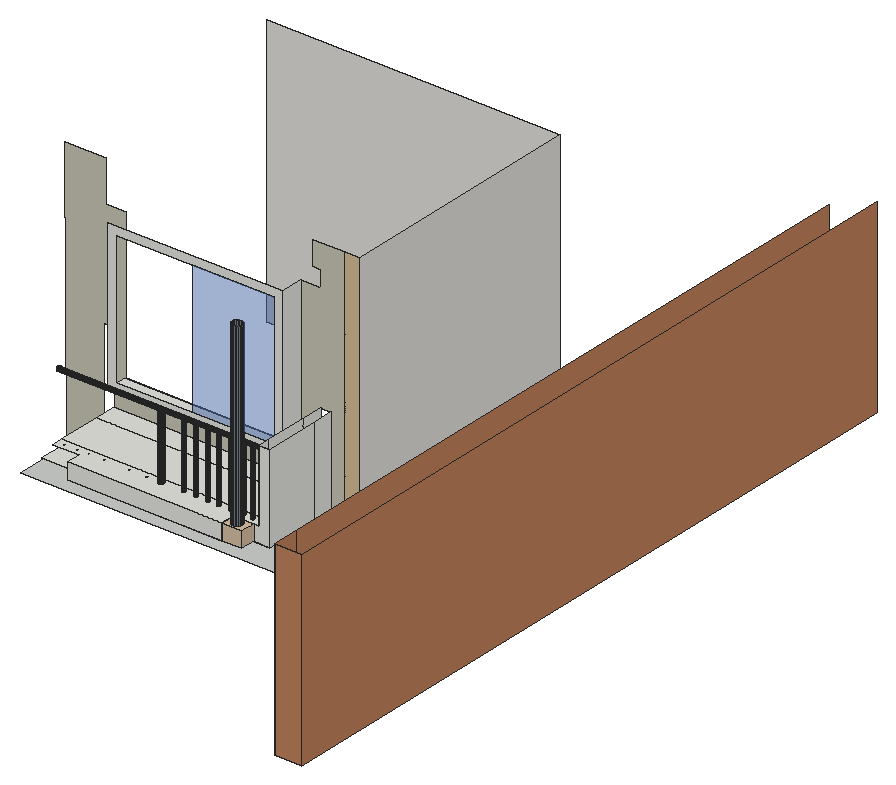
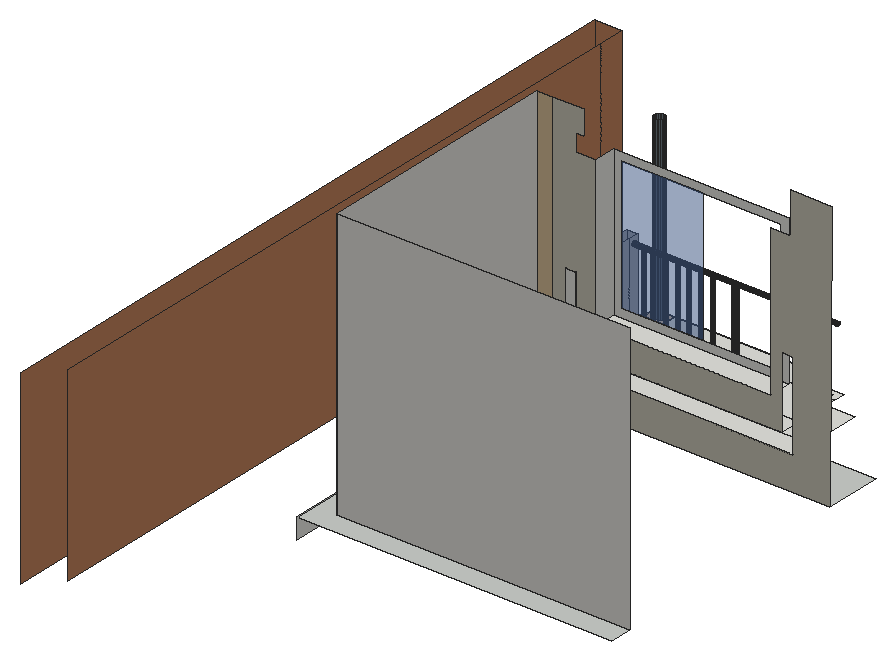
# SketchUp Ruby script. Lengths in inches.
U = 1.inch
M = Sketchup.active_model
def pt(a) = Geom::Point3d.new(a.map { |v| v * U })
def face(e, loops, mat)
  f = e.add_face(loops[0].map { |a| pt(a) })
  loops[1..].each { |l| e.add_face(l.map { |a| pt(a) }).erase! }
  f.material = f.back_material = mat if mat
  f
end
# faces: each face lists its corners as indices into pts; further lists are holes
def faces(e, pts, list, mat = nil) = list.each { |f| face(e, (f[0].is_a?(Array) ? f : [f]).map { |l| l.map { |i| pts[i] } }, mat) }
# xy, xz, yz: faces in a plane at the given z, y or x. An outline is a flat list of corners, or four numbers for a rectangle; further outlines are holes
def ring(l) = l.size == 4 ? [[l[0], l[1]], [l[2], l[1]], [l[2], l[3]], [l[0], l[3]]] : l.each_slice(2).to_a
def flat(e, list, mat, &to3) = list.each { |f| face(e, (f[0].is_a?(Array) ? f : [f]).map { |l| ring(l).map { |u, v| to3.(u, v) } }, mat) }
def xy(e, z, list, mat = nil) = flat(e, list, mat) { |x, y| [x, y, z] }
def xz(e, y, list, mat = nil) = flat(e, list, mat) { |x, z| [x, y, z] }
def yz(e, x, list, mat = nil) = flat(e, list, mat) { |y, z| [x, y, z] }
def lines(e, pts, list) = list.each { |a, b| e.add_line(pt(pts[a]), pt(pts[b])) }
# prism: a flat outline (further loops are holes) pulled along v
def prism(e, loops, v, mat = nil)
  f = face(e, loops, mat); d = Geom::Vector3d.new(v.map { |x| x * U })
  f.pushpull(f.normal.samedirection?(d) ? d.length : -d.length)
end
def box(e, o, s, mat = nil) = prism(e, [[o, [o[0] + s[0], o[1], o[2]], [o[0] + s[0], o[1] + s[1], o[2]], [o[0], o[1] + s[1], o[2]]]], [0, 0, s[2]], mat)
def at(x, y, z, deg = 0) = Geom::Transformation.translation(pt([x, y, z])) * Geom::Transformation.rotation(ORIGIN, Z_AXIS, deg.degrees)
def axes(o, x, y, z) = Geom::Transformation.new([*x, 0, *y, 0, *z, 0, *pt(o).to_a, 1])
def part(name) = M.definitions.add(name)
# library, detail: a bought-in or finely detailed component or shape, given as its bounding box
def library(name, o, s) = part(name).tap { |d| box(d.entities, o, s) }
def detail(e, o, s) = box(e.add_group.entities, o, s)
def put(e, d, t, mat = nil) = e.add_instance(d, t).tap { |i| i.material = mat if mat }
def group(e, t, mat = nil) = e.add_group.tap { |g| g.transformation = t; g.material = mat if mat }.entities
root = M.entities
M.materials.add("[Basic Tile]").color = [203, 206, 202]
M.materials.add("[Formica Beige]").color = [211, 187, 149]
M.materials.add("[Formica Graystone]").color = [198, 194, 180]
M.materials.add("[Formica Laminate Dark]").color = [50, 53, 60]
M.materials.add("[Formica Laminate Light]").color = [213, 189, 164]
M.materials.add("[Formica Speckled Grey]").color = [112, 125, 132]
M.materials.add("[Terrazzo Tile Accent]").color = [224, 221, 217]
M.materials.add("[Translucent Glass Blue]").color = [85, 126, 201]
M.materials["[Translucent Glass Blue]"].alpha = 0.5
M.materials.add("[Wood Veneer 02]").color = [190, 128, 91]
xy(root,9,[[271.94,88.35,402.13,114.1],[402.13,88.35,411.85,88.35,411.85,235.11,271.94,235.11,271.94,225.39,402.13,225.39]],"[Basic Tile]")
xy(root,24.1875,[[304.9375,73.57,304.9375,80.01,288.3125,80.01,288.3125,104.39,389.375,104.39,389.375,80.01,373.41,80.01,373.41,73.57],[288.3125,104.39,389.375,114.1]])
xy(root,24.1875,[[373.41,73.57,382.25,80.01]],"[Formica Laminate Light]")
xy(root,31.3,[[[304.9375,73.57,373.41,73.57,373.41,80.01,384.76,80.01,384.76,84.92,293.16,84.92,293.16,80.01,304.9375,80.01],[339.03,81.65,338.7,81.69,338.4,81.82,338.14,82.02,337.94,82.27,337.82,82.58,337.78,82.9,337.82,83.22,337.94,83.52,338.14,83.78,338.4,83.98,338.7,84.11,339.03,84.15,339.35,84.11,339.65,83.98,339.91,83.78,340.11,83.52,340.23,83.22,340.28,82.9,340.23,82.58,340.11,82.27,339.91,82.02,339.65,81.82,339.35,81.69],[349.03,81.89,348.85,81.92,348.68,81.98,348.54,82.09,348.43,82.24,348.36,82.4,348.34,82.58,348.36,82.76,348.43,82.92,348.54,83.07,348.68,83.18,348.85,83.24,349.03,83.27,349.21,83.24,349.37,83.18,349.51,83.07,349.625,82.92,349.69,82.76,349.72,82.58,349.69,82.4,349.625,82.24,349.51,82.09,349.37,81.98,349.21,81.92],[379.9,81.89,379.73,81.92,379.56,81.98,379.42,82.09,379.31,82.24,379.24,82.4,379.22,82.58,379.24,82.76,379.31,82.92,379.42,83.07,379.56,83.18,379.73,83.24,379.9,83.27,380.08,83.24,380.25,83.18,380.39,83.07,380.5,82.92,380.57,82.76,380.59,82.58,380.57,82.4,380.5,82.24,380.39,82.09,380.25,81.98,380.08,81.92],[354.6875,81.89,354.51,81.92,354.35,81.98,354.2,82.09,354.09,82.24,354.02,82.4,354,82.58,354.02,82.76,354.09,82.92,354.2,83.07,354.35,83.18,354.51,83.24,354.6875,83.27,354.87,83.24,355.03,83.18,355.18,83.07,355.28,82.92,355.35,82.76,355.375,82.58,355.35,82.4,355.28,82.24,355.18,82.09,355.03,81.98,354.87,81.92],[375.8125,81.89,375.64,81.92,375.47,81.98,375.33,82.09,375.22,82.24,375.15,82.4,375.125,82.58,375.15,82.76,375.22,82.92,375.33,83.07,375.47,83.18,375.64,83.24,375.8125,83.27,375.99,83.24,376.16,83.18,376.3,83.07,376.41,82.92,376.48,82.76,376.5,82.58,376.48,82.4,376.41,82.24,376.3,82.09,376.16,81.98,375.99,81.92],[359.9375,81.89,359.76,81.92,359.6,81.98,359.45,82.09,359.34,82.24,359.27,82.4,359.25,82.58,359.27,82.76,359.34,82.92,359.45,83.07,359.6,83.18,359.76,83.24,359.9375,83.27,360.12,83.24,360.28,83.18,360.43,83.07,360.53,82.92,360.6,82.76,360.625,82.58,360.6,82.4,360.53,82.24,360.43,82.09,360.28,81.98,360.12,81.92],[370.25,81.89,370.07,81.92,369.91,81.98,369.77,82.09,369.66,82.24,369.59,82.4,369.5625,82.58,369.59,82.76,369.66,82.92,369.77,83.07,369.91,83.18,370.07,83.24,370.25,83.27,370.43,83.24,370.6,83.18,370.74,83.07,370.85,82.92,370.92,82.76,370.9375,82.58,370.92,82.4,370.85,82.24,370.74,82.09,370.6,81.98,370.43,81.92],[364.8125,81.89,364.64,81.92,364.47,81.98,364.33,82.09,364.22,82.24,364.15,82.4,364.125,82.58,364.15,82.76,364.22,82.92,364.33,83.07,364.47,83.18,364.64,83.24,364.8125,83.27,364.99,83.24,365.16,83.18,365.3,83.07,365.41,82.92,365.48,82.76,365.5,82.58,365.48,82.4,365.41,82.24,365.3,82.09,365.16,81.98,364.99,81.92],[332.6875,81.89,332.51,81.92,332.35,81.98,332.2,82.09,332.09,82.24,332.02,82.4,332,82.58,332.02,82.76,332.09,82.92,332.2,83.07,332.35,83.18,332.51,83.24,332.6875,83.27,332.87,83.24,333.03,83.18,333.18,83.07,333.28,82.92,333.35,82.76,333.375,82.58,333.35,82.4,333.28,82.24,333.18,82.09,333.03,81.98,332.87,81.92],[296.0625,81.89,295.89,81.92,295.72,81.98,295.58,82.09,295.47,82.24,295.4,82.4,295.375,82.58,295.4,82.76,295.47,82.92,295.58,83.07,295.72,83.18,295.89,83.24,296.0625,83.27,296.24,83.24,296.41,83.18,296.55,83.07,296.66,82.92,296.73,82.76,296.75,82.58,296.73,82.4,296.66,82.24,296.55,82.09,296.41,81.98,296.24,81.92],[325.0625,81.89,324.89,81.92,324.72,81.98,324.58,82.09,324.47,82.24,324.4,82.4,324.375,82.58,324.4,82.76,324.47,82.92,324.58,83.07,324.72,83.18,324.89,83.24,325.0625,83.27,325.24,83.24,325.41,83.18,325.55,83.07,325.66,82.92,325.73,82.76,325.75,82.58,325.73,82.4,325.66,82.24,325.55,82.09,325.41,81.98,325.24,81.92],[301.8125,81.89,301.64,81.92,301.47,81.98,301.33,82.09,301.22,82.24,301.15,82.4,301.125,82.58,301.15,82.76,301.22,82.92,301.33,83.07,301.47,83.18,301.64,83.24,301.8125,83.27,301.99,83.24,302.16,83.18,302.3,83.07,302.41,82.92,302.48,82.76,302.5,82.58,302.48,82.4,302.41,82.24,302.3,82.09,302.16,81.98,301.99,81.92],[318.5625,81.89,318.39,81.92,318.22,81.98,318.08,82.09,317.97,82.24,317.9,82.4,317.875,82.58,317.9,82.76,317.97,82.92,318.08,83.07,318.22,83.18,318.39,83.24,318.5625,83.27,318.74,83.24,318.91,83.18,319.05,83.07,319.16,82.92,319.23,82.76,319.25,82.58,319.23,82.4,319.16,82.24,319.05,82.09,318.91,81.98,318.74,81.92],[307.125,81.89,306.95,81.92,306.78,81.98,306.64,82.09,306.53,82.24,306.46,82.4,306.4375,82.58,306.46,82.76,306.53,82.92,306.64,83.07,306.78,83.18,306.95,83.24,307.125,83.27,307.3,83.24,307.47,83.18,307.61,83.07,307.72,82.92,307.79,82.76,307.8125,82.58,307.79,82.4,307.72,82.24,307.61,82.09,307.47,81.98,307.3,81.92],[313.75,81.89,313.57,81.92,313.41,81.98,313.27,82.09,313.16,82.24,313.09,82.4,313.0625,82.58,313.09,82.76,313.16,82.92,313.27,83.07,313.41,83.18,313.57,83.24,313.75,83.27,313.93,83.24,314.1,83.18,314.24,83.07,314.35,82.92,314.42,82.76,314.4375,82.58,314.42,82.4,314.35,82.24,314.24,82.09,314.1,81.98,313.93,81.92]],[377.92,74.4375,377.32,74.44,376.74,74.61,376.22,74.92,375.8,75.35,375.5,75.875,375.35,76.46,375.36,77.0625,375.52,77.64,375.83,78.16,376.26,78.58,376.79,78.88,377.375,79.03,377.98,79.02,378.56,78.86,379.08,78.55,379.5,78.12,379.8,77.59,379.94,77.01,379.9375,76.4,379.77,75.82,379.47,75.3,379.03,74.88,378.51,74.59],[339.03,81.65,338.7,81.69,338.4,81.82,338.14,82.02,337.94,82.27,337.82,82.58,337.78,82.9,337.82,83.22,337.94,83.52,338.14,83.78,338.4,83.98,338.7,84.11,339.03,84.15,339.35,84.11,339.65,83.98,339.91,83.78,340.11,83.52,340.23,83.22,340.28,82.9,340.23,82.58,340.11,82.27,339.91,82.02,339.65,81.82,339.35,81.69],[349.03,81.89,348.85,81.92,348.68,81.98,348.54,82.09,348.43,82.24,348.36,82.4,348.34,82.58,348.36,82.76,348.43,82.92,348.54,83.07,348.68,83.18,348.85,83.24,349.03,83.27,349.21,83.24,349.37,83.18,349.51,83.07,349.625,82.92,349.69,82.76,349.72,82.58,349.69,82.4,349.625,82.24,349.51,82.09,349.37,81.98,349.21,81.92],[354.6875,81.89,354.51,81.92,354.35,81.98,354.2,82.09,354.09,82.24,354.02,82.4,354,82.58,354.02,82.76,354.09,82.92,354.2,83.07,354.35,83.18,354.51,83.24,354.6875,83.27,354.87,83.24,355.03,83.18,355.18,83.07,355.28,82.92,355.35,82.76,355.375,82.58,355.35,82.4,355.28,82.24,355.18,82.09,355.03,81.98,354.87,81.92],
  [359.9375,81.89,359.76,81.92,359.6,81.98,359.45,82.09,359.34,82.24,359.27,82.4,359.25,82.58,359.27,82.76,359.34,82.92,359.45,83.07,359.6,83.18,359.76,83.24,359.9375,83.27,360.12,83.24,360.28,83.18,360.43,83.07,360.53,82.92,360.6,82.76,360.625,82.58,360.6,82.4,360.53,82.24,360.43,82.09,360.28,81.98,360.12,81.92],[364.8125,81.89,364.64,81.92,364.47,81.98,364.33,82.09,364.22,82.24,364.15,82.4,364.125,82.58,364.15,82.76,364.22,82.92,364.33,83.07,364.47,83.18,364.64,83.24,364.8125,83.27,364.99,83.24,365.16,83.18,365.3,83.07,365.41,82.92,365.48,82.76,365.5,82.58,365.48,82.4,365.41,82.24,365.3,82.09,365.16,81.98,364.99,81.92],[370.25,81.89,370.07,81.92,369.91,81.98,369.77,82.09,369.66,82.24,369.59,82.4,369.5625,82.58,369.59,82.76,369.66,82.92,369.77,83.07,369.91,83.18,370.07,83.24,370.25,83.27,370.43,83.24,370.6,83.18,370.74,83.07,370.85,82.92,370.92,82.76,370.9375,82.58,370.92,82.4,370.85,82.24,370.74,82.09,370.6,81.98,370.43,81.92],[375.8125,81.89,375.64,81.92,375.47,81.98,375.33,82.09,375.22,82.24,375.15,82.4,375.125,82.58,375.15,82.76,375.22,82.92,375.33,83.07,375.47,83.18,375.64,83.24,375.8125,83.27,375.99,83.24,376.16,83.18,376.3,83.07,376.41,82.92,376.48,82.76,376.5,82.58,376.48,82.4,376.41,82.24,376.3,82.09,376.16,81.98,375.99,81.92],[379.9,81.89,379.73,81.92,379.56,81.98,379.42,82.09,379.31,82.24,379.24,82.4,379.22,82.58,379.24,82.76,379.31,82.92,379.42,83.07,379.56,83.18,379.73,83.24,379.9,83.27,380.08,83.24,380.25,83.18,380.39,83.07,380.5,82.92,380.57,82.76,380.59,82.58,380.57,82.4,380.5,82.24,380.39,82.09,380.25,81.98,380.08,81.92],
  [293.16,84.92,384.76,104.39],[293.16,104.39,384.76,114.1]])
xy(root,31.3,[[[373.41,73.57,382.25,80.01],[377.92,74.4375,377.32,74.44,376.74,74.61,376.22,74.92,375.8,75.35,375.5,75.875,375.35,76.46,375.36,77.0625,375.52,77.64,375.83,78.16,376.26,78.58,376.79,78.88,377.375,79.03,377.98,79.02,378.56,78.86,379.08,78.55,379.5,78.12,379.8,77.59,379.94,77.01,379.9375,76.4,379.77,75.82,379.47,75.3,379.03,74.88,378.51,74.59]]],"[Formica Laminate Light]")
xy(root,44.62,[[298,104.39,375.8125,114.1]])
xy(root,60.05,[[339.03,81.65,339.35,81.69,339.65,81.82,339.91,82.02,340.11,82.27,340.23,82.58,340.28,82.9,340.23,83.22,340.11,83.52,339.91,83.78,339.65,83.98,339.35,84.11,339.03,84.15,338.7,84.11,338.4,83.98,338.14,83.78,337.94,83.52,337.82,83.22,337.78,82.9,337.82,82.58,337.94,82.27,338.14,82.02,338.4,81.82,338.7,81.69]],"[Formica Laminate Dark]")
xy(root,60.11,[[364.8125,81.89,364.99,81.92,365.16,81.98,365.3,82.09,365.41,82.24,365.48,82.4,365.5,82.58,365.48,82.76,365.41,82.92,365.3,83.07,365.16,83.18,364.99,83.24,364.8125,83.27,364.64,83.24,364.47,83.18,364.33,83.07,364.22,82.92,364.15,82.76,364.125,82.58,364.15,82.4,364.22,82.24,364.33,82.09,364.47,81.98,364.64,81.92]])
xy(root,60.36,[[370.25,81.89,370.43,81.92,370.6,81.98,370.74,82.09,370.85,82.24,370.92,82.4,370.9375,82.58,370.92,82.76,370.85,82.92,370.74,83.07,370.6,83.18,370.43,83.24,370.25,83.27,370.07,83.24,369.91,83.18,369.77,83.07,369.66,82.92,369.59,82.76,369.5625,82.58,369.59,82.4,369.66,82.24,369.77,82.09,369.91,81.98,370.07,81.92],[375.8125,81.89,375.99,81.92,376.16,81.98,376.3,82.09,376.41,82.24,376.48,82.4,376.5,82.58,376.48,82.76,376.41,82.92,376.3,83.07,376.16,83.18,375.99,83.24,375.8125,83.27,375.64,83.24,375.47,83.18,375.33,83.07,375.22,82.92,375.15,82.76,375.125,82.58,375.15,82.4,375.22,82.24,375.33,82.09,375.47,81.98,375.64,81.92]])
xy(root,60.42,[[354.6875,81.89,354.87,81.92,355.03,81.98,355.18,82.09,355.28,82.24,355.35,82.4,355.375,82.58,355.35,82.76,355.28,82.92,355.18,83.07,355.03,83.18,354.87,83.24,354.6875,83.27,354.51,83.24,354.35,83.18,354.2,83.07,354.09,82.92,354.02,82.76,354,82.58,354.02,82.4,354.09,82.24,354.2,82.09,354.35,81.98,354.51,81.92],[379.9,81.89,380.08,81.92,380.25,81.98,380.39,82.09,380.5,82.24,380.57,82.4,380.59,82.58,380.57,82.76,380.5,82.92,380.39,83.07,380.25,83.18,380.08,83.24,379.9,83.27,379.73,83.24,379.56,83.18,379.42,83.07,379.31,82.92,379.24,82.76,379.22,82.58,379.24,82.4,379.31,82.24,379.42,82.09,379.56,81.98,379.73,81.92]])
xy(root,60.8,[[349.03,81.89,349.21,81.92,349.37,81.98,349.51,82.09,349.625,82.24,349.69,82.4,349.72,82.58,349.69,82.76,349.625,82.92,349.51,83.07,349.37,83.18,349.21,83.24,349.03,83.27,348.85,83.24,348.68,83.18,348.54,83.07,348.43,82.92,348.36,82.76,348.34,82.58,348.36,82.4,348.43,82.24,348.54,82.09,348.68,81.98,348.85,81.92]])
xy(root,60.8125,[[359.9375,81.89,360.12,81.92,360.28,81.98,360.43,82.09,360.53,82.24,360.6,82.4,360.625,82.58,360.6,82.76,360.53,82.92,360.43,83.07,360.28,83.18,360.12,83.24,359.9375,83.27,359.76,83.24,359.6,83.18,359.45,83.07,359.34,82.92,359.27,82.76,359.25,82.58,359.27,82.4,359.34,82.24,359.45,82.09,359.6,81.98,359.76,81.92]])
xz(root,0,[[455.72,0,467.51,84]],"[Wood Veneer 02]")
xz(root,73.57,[[304.9375,24.1875,373.41,31.3]])
xz(root,73.57,[[373.41,24.1875,382.25,31.3]],"[Formica Laminate Light]")
xz(root,80.01,[[373.41,24.1875,382.25,31.3],[382.25,24.1875,389.375,24.1875,389.375,63.125,384.76,63.125,384.76,31.3,382.25,31.3]])
xz(root,104.39,[[[298,44.62,375.8125,110.81],[301.61,48.23,372.21,107.2]]])
xz(root,104.39,[[335.97,48.23,372.21,107.2]],"[Translucent Glass Blue]")
xz(root,114.1,[[395.49,9,402.13,129]],"[Formica Beige]")
xz(root,114.1,[[[271.94,9,395.49,9,395.49,129,381.1875,129,381.1875,118.3125,384.875,118.3125,384.875,110.81,375.8125,110.81,375.8125,44.62,298,44.62,298,110.81,289.1875,110.81,289.1875,129,270.97,129],[288.3125,24.1875,288.3125,63.125,293.16,63.125,293.16,31.3,384.76,31.3,384.76,63.125,389.375,63.125,389.375,24.1875]]],"[Formica Graystone]")
xz(root,225.39,[[271.94,9,402.13,129]],"[Terrazzo Tile Accent]")
yz(root,373.41,[[73.57,24.1875,80.01,31.3]])
yz(root,375.8125,[[104.39,44.62,114.1,110.81]])
yz(root,382.25,[[73.57,24.1875,80.01,31.3]],"[Formica Laminate Light]")
yz(root,384.76,[[[80.01,31.3,84.92,63.125],[82.67,59.79,82.88,59.82,83.08,59.9,83.25,60.03,83.375,60.2,83.46,60.39,83.48,60.6,83.46,60.8125,83.375,61.01,83.25,61.18,83.08,61.31,82.88,61.39,82.67,61.42,82.46,61.39,82.26,61.31,82.1,61.18,81.97,61.01,81.89,60.8125,81.86,60.6,81.89,60.39,81.97,60.2,82.1,60.03,82.26,59.9,82.46,59.82]],[84.92,31.3,104.39,63.125],[104.39,31.3,114.1,63.125],[82.67,59.79,82.88,59.82,83.08,59.9,83.25,60.03,83.375,60.2,83.46,60.39,83.48,60.6,83.46,60.8125,83.375,61.01,83.25,61.18,83.08,61.31,82.88,61.39,82.67,61.42,82.46,61.39,82.26,61.31,82.1,61.18,81.97,61.01,81.89,60.8125,81.86,60.6,81.89,60.39,81.97,60.2,82.1,60.03,82.26,59.9,82.46,59.82]])
yz(root,389.375,[[80.01,24.1875,104.39,63.125],[104.39,24.1875,114.1,63.125]])
yz(root,402.13,[[114.1,9,225.39,129]],"[Terrazzo Tile Accent]")
yz(root,411.85,[[88.35,0,235.11,9]])
yz(root,455.72,[[0,0,11.79,84],[11.79,0,307.53,84]],"[Wood Veneer 02]")
yz(root,467.51,[[0,0,319.32,84]],"[Wood Veneer 02]")
p = [[376.74,74.61,31.3],[377.32,74.44,31.3],[377.32,74.44,110.81],[376.74,74.61,110.81],[377.92,74.4375,31.3],[377.92,74.4375,110.81],
  [378.51,74.59,31.3],[378.51,74.59,110.81],[376.22,74.92,31.3],[376.22,74.92,110.81],[379.03,74.88,31.3],[379.03,74.88,110.81],
  [375.8,75.35,31.3],[375.8,75.35,110.81],[379.47,75.3,31.3],[379.47,75.3,110.81],[375.5,75.875,31.3],[375.5,75.875,110.81],
  [379.77,75.82,31.3],[379.77,75.82,110.81],[379.9375,76.4,31.3],[379.9375,76.4,110.81],[375.35,76.46,31.3],[375.35,76.46,110.81],
  [379.94,77.01,31.3],[379.94,77.01,110.81],[375.36,77.0625,31.3],[375.36,77.0625,110.81],[379.8,77.59,31.3],[379.8,77.59,110.81],
  [375.52,77.64,31.3],[375.52,77.64,110.81],[375.83,78.16,31.3],[375.83,78.16,110.81],[379.5,78.12,31.3],[379.5,78.12,110.81],
  [379.08,78.55,31.3],[379.08,78.55,110.81],[376.26,78.58,31.3],[376.26,78.58,110.81],[376.79,78.88,31.3],[376.79,78.88,110.81],
  [378.56,78.86,31.3],[378.56,78.86,110.81],[377.375,79.03,31.3],[377.375,79.03,110.81],[377.98,79.02,31.3],[377.98,79.02,110.81],
  [338.7,81.69,31.3],[339.03,81.65,31.3],[339.03,81.65,60.05],[338.7,81.69,60.05],[339.35,81.69,31.3],[339.35,81.69,60.05],
  [338.4,81.82,31.3],[338.4,81.82,60.05],[339.65,81.82,31.3],[339.65,81.82,60.05],[338.14,82.02,31.3],[338.14,82.02,60.05],
  [339.91,82.02,31.3],[339.91,82.02,60.05],[348.68,81.98,31.3],[348.85,81.92,31.3],[348.85,81.92,60.8],[348.68,81.98,60.8],
  [349.03,81.89,31.3],[349.03,81.89,60.8],[349.21,81.92,31.3],[349.21,81.92,60.8],[349.37,81.98,31.3],[349.37,81.98,60.8],
  [354.35,81.98,31.3],[354.51,81.92,31.3],[354.51,81.92,60.42],[354.35,81.98,60.42],[354.6875,81.89,31.3],[354.6875,81.89,60.42],
  [354.87,81.92,31.3],[354.87,81.92,60.42],[355.03,81.98,31.3],[355.03,81.98,60.42],[359.6,81.98,31.3],[359.76,81.92,31.3],
  [359.76,81.92,60.8125],[359.6,81.98,60.8125],[359.9375,81.89,31.3],[359.9375,81.89,60.8125],[360.12,81.92,31.3],[360.12,81.92,60.8125],
  [360.28,81.98,31.3],[360.28,81.98,60.8125],[364.47,81.98,31.3],[364.64,81.92,31.3],[364.64,81.92,60.11],[364.47,81.98,60.11],
  [364.8125,81.89,31.3],[364.8125,81.89,60.11],[364.99,81.92,31.3],[364.99,81.92,60.11],[365.16,81.98,31.3],[365.16,81.98,60.11],
  [369.91,81.98,31.3],[370.07,81.92,31.3],[370.07,81.92,60.36],[369.91,81.98,60.36],[370.25,81.89,31.3],[370.25,81.89,60.36],
  [370.43,81.92,31.3],[370.43,81.92,60.36],[370.6,81.98,31.3],[370.6,81.98,60.36],[375.47,81.98,31.3],[375.64,81.92,31.3],
  [375.64,81.92,60.36],[375.47,81.98,60.36],[375.8125,81.89,31.3],[375.8125,81.89,60.36],[375.99,81.92,31.3],[375.99,81.92,60.36],
  [376.16,81.98,31.3],[376.16,81.98,60.36],[379.56,81.98,31.3],[379.73,81.92,31.3],[379.73,81.92,60.42],[379.56,81.98,60.42],
  [379.9,81.89,31.3],[379.9,81.89,60.42],[380.08,81.92,31.3],[380.08,81.92,60.42],[380.25,81.98,31.3],[380.25,81.98,60.42],
  [337.94,82.27,31.3],[337.94,82.27,60.05],[340.11,82.27,31.3],[340.11,82.27,60.05],[348.54,82.09,31.3],[348.54,82.09,60.8],
  [349.51,82.09,31.3],[349.51,82.09,60.8],[354.2,82.09,31.3],[354.2,82.09,60.42],[355.18,82.09,31.3],[355.18,82.09,60.42],
  [359.45,82.09,31.3],[359.45,82.09,60.8125],[360.43,82.09,31.3],[360.43,82.09,60.8125],[364.33,82.09,31.3],[364.33,82.09,60.11],
  [365.3,82.09,31.3],[365.3,82.09,60.11],[369.77,82.09,31.3],[369.77,82.09,60.36],[370.74,82.09,31.3],[370.74,82.09,60.36],
  [375.33,82.09,31.3],[375.33,82.09,60.36],[376.3,82.09,31.3],[376.3,82.09,60.36],[379.42,82.09,31.3],[379.42,82.09,60.42],
  [380.39,82.09,31.3],[380.39,82.09,60.42],[348.43,82.24,31.3],[348.43,82.24,60.8],[349.625,82.24,31.3],[349.625,82.24,60.8],
  [354.09,82.24,31.3],[354.09,82.24,60.42],[355.28,82.24,31.3],[355.28,82.24,60.42],[359.34,82.24,31.3],[359.34,82.24,60.8125],
  [360.53,82.24,31.3],[360.53,82.24,60.8125],[364.22,82.24,31.3],[364.22,82.24,60.11],[365.41,82.24,31.3],[365.41,82.24,60.11],
  [369.66,82.24,31.3],[369.66,82.24,60.36],[370.85,82.24,31.3],[370.85,82.24,60.36],[375.22,82.24,31.3],[375.22,82.24,60.36],
  [376.41,82.24,31.3],[376.41,82.24,60.36],[379.31,82.24,31.3],[379.31,82.24,60.42],[380.5,82.24,31.3],[380.5,82.24,60.42],
  [348.36,82.4,31.3],[348.36,82.4,60.8],[349.69,82.4,31.3],[349.69,82.4,60.8],[354.02,82.4,31.3],[354.02,82.4,60.42],
  [355.35,82.4,31.3],[355.35,82.4,60.42],[359.27,82.4,31.3],[359.27,82.4,60.8125],[360.6,82.4,31.3],[360.6,82.4,60.8125],
  [364.15,82.4,31.3],[364.15,82.4,60.11],[365.48,82.4,31.3],[365.48,82.4,60.11],[369.59,82.4,31.3],[369.59,82.4,60.36],
  [370.92,82.4,31.3],[370.92,82.4,60.36],[375.15,82.4,31.3],[375.15,82.4,60.36],[376.48,82.4,31.3],[376.48,82.4,60.36],
  [379.24,82.4,31.3],[379.24,82.4,60.42],[380.57,82.4,31.3],[380.57,82.4,60.42],[337.82,82.58,31.3],[337.82,82.58,60.05],
  [340.23,82.58,31.3],[340.23,82.58,60.05],[348.34,82.58,31.3],[348.34,82.58,60.8],[349.72,82.58,31.3],[349.72,82.58,60.8],
  [354,82.58,31.3],[354,82.58,60.42],[355.375,82.58,31.3],[355.375,82.58,60.42],[359.25,82.58,31.3],[359.25,82.58,60.8125],
  [360.625,82.58,31.3],[360.625,82.58,60.8125],[364.125,82.58,31.3],[364.125,82.58,60.11],[365.5,82.58,31.3],[365.5,82.58,60.11],
  [369.5625,82.58,31.3],[369.5625,82.58,60.36],[370.9375,82.58,31.3],[370.9375,82.58,60.36],[375.125,82.58,31.3],[375.125,82.58,60.36],
  [376.5,82.58,31.3],[376.5,82.58,60.36],[379.22,82.58,31.3],[379.22,82.58,60.42],[380.59,82.58,31.3],[380.59,82.58,60.42],
  [337.78,82.9,31.3],[337.78,82.9,60.05],[340.28,82.9,31.3],[340.28,82.9,60.05],[348.36,82.76,31.3],[348.36,82.76,60.8],
  [349.69,82.76,31.3],[349.69,82.76,60.8],[354.02,82.76,31.3],[354.02,82.76,60.42],[355.35,82.76,31.3],[355.35,82.76,60.42],
  [359.27,82.76,31.3],[359.27,82.76,60.8125],[360.6,82.76,31.3],[360.6,82.76,60.8125],[364.15,82.76,31.3],[364.15,82.76,60.11],
  [365.48,82.76,31.3],[365.48,82.76,60.11],[369.59,82.76,31.3],[369.59,82.76,60.36],[370.92,82.76,31.3],[370.92,82.76,60.36],
  [375.15,82.76,31.3],[375.15,82.76,60.36],[376.48,82.76,31.3],[376.48,82.76,60.36],[379.24,82.76,31.3],[379.24,82.76,60.42],
  [380.57,82.76,31.3],[380.57,82.76,60.42],[348.43,82.92,31.3],[348.43,82.92,60.8],[349.625,82.92,31.3],[349.625,82.92,60.8],
  [354.09,82.92,31.3],[354.09,82.92,60.42],[355.28,82.92,31.3],[355.28,82.92,60.42],[359.34,82.92,31.3],[359.34,82.92,60.8125],
  [360.53,82.92,31.3],[360.53,82.92,60.8125],[364.22,82.92,31.3],[364.22,82.92,60.11],[365.41,82.92,31.3],[365.41,82.92,60.11],
  [369.66,82.92,31.3],[369.66,82.92,60.36],[370.85,82.92,31.3],[370.85,82.92,60.36],[375.22,82.92,31.3],[375.22,82.92,60.36],
  [376.41,82.92,31.3],[376.41,82.92,60.36],[379.31,82.92,31.3],[379.31,82.92,60.42],[380.5,82.92,31.3],[380.5,82.92,60.42],
  [337.82,83.22,31.3],[337.82,83.22,60.05],[340.23,83.22,31.3],[340.23,83.22,60.05],[348.54,83.07,31.3],[348.54,83.07,60.8],
  [349.51,83.07,31.3],[349.51,83.07,60.8],[354.2,83.07,31.3],[354.2,83.07,60.42],[355.18,83.07,31.3],[355.18,83.07,60.42],
  [359.45,83.07,31.3],[359.45,83.07,60.8125],[360.43,83.07,31.3],[360.43,83.07,60.8125],[364.33,83.07,31.3],[364.33,83.07,60.11],
  [365.3,83.07,31.3],[365.3,83.07,60.11],[369.77,83.07,31.3],[369.77,83.07,60.36],[370.74,83.07,31.3],[370.74,83.07,60.36],
  [375.33,83.07,31.3],[375.33,83.07,60.36],[376.3,83.07,31.3],[376.3,83.07,60.36],[379.42,83.07,31.3],[379.42,83.07,60.42],
  [380.39,83.07,31.3],[380.39,83.07,60.42],[348.68,83.18,31.3],[348.68,83.18,60.8],[349.37,83.18,31.3],[349.37,83.18,60.8],
  [354.35,83.18,31.3],[354.35,83.18,60.42],[355.03,83.18,31.3],[355.03,83.18,60.42],[359.6,83.18,31.3],[359.6,83.18,60.8125],
  [360.28,83.18,31.3],[360.28,83.18,60.8125],[364.47,83.18,31.3],[364.47,83.18,60.11],[365.16,83.18,31.3],[365.16,83.18,60.11],
  [369.91,83.18,31.3],[369.91,83.18,60.36],[370.6,83.18,31.3],[370.6,83.18,60.36],[375.47,83.18,31.3],[375.47,83.18,60.36],
  [376.16,83.18,31.3],[376.16,83.18,60.36],[379.56,83.18,31.3],[379.56,83.18,60.42],[380.25,83.18,31.3],[380.25,83.18,60.42],
  [337.94,83.52,31.3],[337.94,83.52,60.05],[340.11,83.52,31.3],[340.11,83.52,60.05],[348.85,83.24,31.3],[348.85,83.24,60.8],
  [349.03,83.27,31.3],[349.03,83.27,60.8],[349.21,83.24,31.3],[349.21,83.24,60.8],[354.51,83.24,31.3],[354.51,83.24,60.42],
  [354.6875,83.27,31.3],[354.6875,83.27,60.42],[354.87,83.24,31.3],[354.87,83.24,60.42],[359.76,83.24,31.3],[359.76,83.24,60.8125],
  [359.9375,83.27,31.3],[359.9375,83.27,60.8125],[360.12,83.24,31.3],[360.12,83.24,60.8125],[364.64,83.24,31.3],[364.64,83.24,60.11],
  [364.8125,83.27,31.3],[364.8125,83.27,60.11],[364.99,83.24,31.3],[364.99,83.24,60.11],[370.07,83.24,31.3],[370.07,83.24,60.36],
  [370.25,83.27,31.3],[370.25,83.27,60.36],[370.43,83.24,31.3],[370.43,83.24,60.36],[375.64,83.24,31.3],[375.64,83.24,60.36],
  [375.8125,83.27,31.3],[375.8125,83.27,60.36],[375.99,83.24,31.3],[375.99,83.24,60.36],[379.73,83.24,31.3],[379.73,83.24,60.42],
  [379.9,83.27,31.3],[379.9,83.27,60.42],[380.08,83.24,31.3],[380.08,83.24,60.42],[338.14,83.78,31.3],[338.14,83.78,60.05],
  [339.91,83.78,31.3],[339.91,83.78,60.05],[338.4,83.98,31.3],[338.4,83.98,60.05],[339.65,83.98,31.3],[339.65,83.98,60.05],
  [338.7,84.11,31.3],[338.7,84.11,60.05],[339.35,84.11,31.3],[339.35,84.11,60.05],[339.03,84.15,31.3],[339.03,84.15,60.05],
  [384.76,82.46,59.82],[384.76,82.26,59.9],[293.16,82.26,59.9],[293.16,82.46,59.82],[384.76,82.67,59.79],[293.16,82.67,59.79],
  [384.76,82.88,59.82],[293.16,82.88,59.82],[384.76,83.08,59.9],[293.16,83.08,59.9],[384.76,82.1,60.03],[293.16,82.1,60.03],
  [384.76,83.25,60.03],[293.16,83.25,60.03],[384.76,81.97,60.2],[293.16,81.97,60.2],[384.76,83.375,60.2],[293.16,83.375,60.2],
  [384.76,81.89,60.39],[293.16,81.89,60.39],[384.76,83.46,60.39],[293.16,83.46,60.39],[384.76,81.86,60.6],[293.16,81.86,60.6],
  [384.76,83.48,60.6],[293.16,83.48,60.6],[384.76,81.89,60.8125],[293.16,81.89,60.8125],[384.76,83.46,60.8125],[293.16,83.46,60.8125],
  [384.76,83.375,61.01],[293.16,83.375,61.01],[384.76,81.97,61.01],[384.76,82.1,61.18],[293.16,82.1,61.18],[293.16,81.97,61.01],
  [324.76,81.97,61.01],[325.37,81.97,61.01],[384.76,83.25,61.18],[293.16,83.25,61.18],[384.76,82.26,61.31],[293.16,82.26,61.31],
  [384.76,83.08,61.31],[293.16,83.08,61.31],[384.76,82.46,61.39],[293.16,82.46,61.39],[384.76,82.88,61.39],[293.16,82.88,61.39],
  [384.76,82.67,61.42],[293.16,82.67,61.42]]
faces(root,p,[[0,1,2,3],[1,4,5,2],[4,6,7,5],[8,0,3,9],[6,10,11,7],[12,8,9,13],[10,14,15,11],[16,12,13,17],
  [14,18,19,15],[18,20,21,19],[22,16,17,23],[20,24,25,21],[26,22,23,27],[24,28,29,25],[30,26,27,31],[32,30,31,33],
  [28,34,35,29],[34,36,37,35],[38,32,33,39],[40,38,39,41],[36,42,43,37],[44,40,41,45],[42,46,47,43],[46,44,45,47]],"[Formica Speckled Grey]")
faces(root,p,[[48,49,50,51],[49,52,53,50],[54,48,51,55],[52,56,57,53],[58,54,55,59],[56,60,61,57],[62,63,64,65],[63,66,67,64],
  [66,68,69,67],[68,70,71,69],[72,73,74,75],[73,76,77,74],[76,78,79,77],[78,80,81,79],[82,83,84,85],[83,86,87,84],
  [86,88,89,87],[88,90,91,89],[92,93,94,95],[93,96,97,94],[96,98,99,97],[98,100,101,99],[102,103,104,105],[103,106,107,104],
  [106,108,109,107],[108,110,111,109],[112,113,114,115],[113,116,117,114],[116,118,119,117],[118,120,121,119],[122,123,124,125],[123,126,127,124],
  [126,128,129,127],[128,130,131,129],[132,58,59,133],[60,134,135,61],[136,62,65,137],[70,138,139,71],[140,72,75,141],[80,142,143,81],
  [144,82,85,145],[90,146,147,91],[148,92,95,149],[100,150,151,101],[152,102,105,153],[110,154,155,111],[156,112,115,157],[120,158,159,121],
  [160,122,125,161],[130,162,163,131],[164,136,137,165],[138,166,167,139],[168,140,141,169],[142,170,171,143],[172,144,145,173],[146,174,175,147],
  [176,148,149,177],[150,178,179,151],[180,152,153,181],[154,182,183,155],[184,156,157,185],[158,186,187,159],[188,160,161,189],[162,190,191,163],
  [192,164,165,193],[166,194,195,167],[196,168,169,197],[170,198,199,171],[200,172,173,201],[174,202,203,175],[204,176,177,205],[178,206,207,179],
  [208,180,181,209],[182,210,211,183],[212,184,185,213],[186,214,215,187],[216,188,189,217],[190,218,219,191],[220,132,133,221],[134,222,223,135],
  [224,192,193,225],[194,226,227,195],[228,196,197,229],[198,230,231,199],[232,200,201,233],[202,234,235,203],[236,204,205,237],[206,238,239,207],
  [240,208,209,241],[210,242,243,211],[244,212,213,245],[214,246,247,215],[248,216,217,249],[218,250,251,219],[252,220,221,253],[222,254,255,223],
  [256,224,225,257],[226,258,259,227],[260,228,229,261],[230,262,263,231],[264,232,233,265],[234,266,267,235],[268,236,237,269],[238,270,271,239],
  [272,240,241,273],[242,274,275,243],[276,244,245,277],[246,278,279,247],[280,248,249,281],[250,282,283,251],[284,256,257,285],[258,286,287,259],
  [288,260,261,289],[262,290,291,263],[292,264,265,293],[266,294,295,267],[296,268,269,297],[270,298,299,271],[300,272,273,301],[274,302,303,275],
  [304,276,277,305],[278,306,307,279],[308,280,281,309],[282,310,311,283],[312,252,253,313],[254,314,315,255],[316,284,285,317],[286,318,319,287],
  [320,288,289,321],[290,322,323,291],[324,292,293,325],[294,326,327,295],[328,296,297,329],[298,330,331,299],[332,300,301,333],[302,334,335,303],
  [336,304,305,337],[306,338,339,307],[340,308,309,341],[310,342,343,311],[344,316,317,345],[318,346,347,319],[348,320,321,349],[322,350,351,323],
  [352,324,325,353],[326,354,355,327],[356,328,329,357],[330,358,359,331],[360,332,333,361],[334,362,363,335],[364,336,337,365],[338,366,367,339],
  [368,340,341,369],[342,370,371,343],[372,312,313,373],[314,374,375,315],[376,344,345,377],[378,376,377,379],[380,378,379,381],[346,380,381,347],
  [382,348,349,383],[384,382,383,385],[386,384,385,387],[350,386,387,351],[388,352,353,389],[390,388,389,391],[392,390,391,393],[354,392,393,355],
  [394,356,357,395],[396,394,395,397],[398,396,397,399],[358,398,399,359],[400,360,361,401],[402,400,401,403],[404,402,403,405],[362,404,405,363],
  [406,364,365,407],[408,406,407,409],[410,408,409,411],[366,410,411,367],[412,368,369,413],[414,412,413,415],[416,414,415,417],[370,416,417,371],
  [418,372,373,419],[374,420,421,375],[422,418,419,423],[420,424,425,421],[426,422,423,427],[424,428,429,425],[430,426,427,431],[428,430,431,429],
  [432,433,434,435],[436,432,435,437],[438,436,437,439],[440,438,439,441],[433,442,443,434],[444,440,441,445],[442,446,447,443],[448,444,445,449],
  [446,450,451,447],[452,448,449,453],[450,454,455,451],[456,452,453,457],[454,458,459,455],[460,456,457,461],[462,460,461,463],[464,465,466,467,468,469],
  [470,462,463,471],[465,472,473,466],[474,470,471,475],[472,476,477,473],[478,474,475,479],[476,480,481,477],[480,478,479,481]],"[Formica Laminate Dark]")
